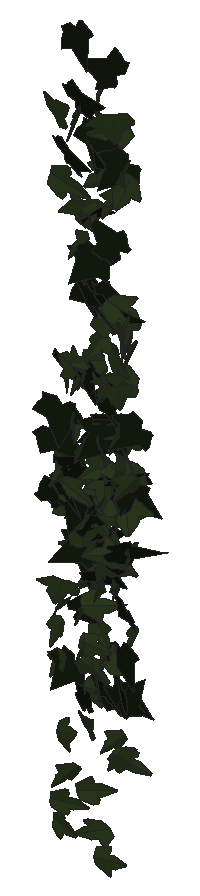
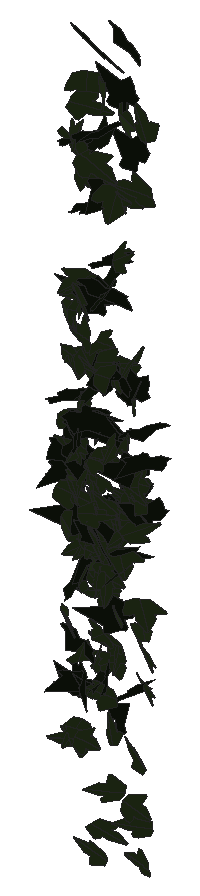
# SketchUp Ruby script. Lengths in inches.
U = 1.inch
M = Sketchup.active_model
def pt(a) = Geom::Point3d.new(a.map { |v| v * U })
def face(e, loops, mat)
  f = e.add_face(loops[0].map { |a| pt(a) })
  loops[1..].each { |l| e.add_face(l.map { |a| pt(a) }).erase! }
  f.material = f.back_material = mat if mat
  f
end
# faces: each face lists its corners as indices into pts; further lists are holes
def faces(e, pts, list, mat = nil) = list.each { |f| face(e, (f[0].is_a?(Array) ? f : [f]).map { |l| l.map { |i| pts[i] } }, mat) }
# xy, xz, yz: faces in a plane at the given z, y or x. An outline is a flat list of corners, or four numbers for a rectangle; further outlines are holes
def ring(l) = l.size == 4 ? [[l[0], l[1]], [l[2], l[1]], [l[2], l[3]], [l[0], l[3]]] : l.each_slice(2).to_a
def flat(e, list, mat, &to3) = list.each { |f| face(e, (f[0].is_a?(Array) ? f : [f]).map { |l| ring(l).map { |u, v| to3.(u, v) } }, mat) }
def xy(e, z, list, mat = nil) = flat(e, list, mat) { |x, y| [x, y, z] }
def xz(e, y, list, mat = nil) = flat(e, list, mat) { |x, z| [x, y, z] }
def yz(e, x, list, mat = nil) = flat(e, list, mat) { |y, z| [x, y, z] }
def lines(e, pts, list) = list.each { |a, b| e.add_line(pt(pts[a]), pt(pts[b])) }
# prism: a flat outline (further loops are holes) pulled along v
def prism(e, loops, v, mat = nil)
  f = face(e, loops, mat); d = Geom::Vector3d.new(v.map { |x| x * U })
  f.pushpull(f.normal.samedirection?(d) ? d.length : -d.length)
end
def box(e, o, s, mat = nil) = prism(e, [[o, [o[0] + s[0], o[1], o[2]], [o[0] + s[0], o[1] + s[1], o[2]], [o[0], o[1] + s[1], o[2]]]], [0, 0, s[2]], mat)
def at(x, y, z, deg = 0) = Geom::Transformation.translation(pt([x, y, z])) * Geom::Transformation.rotation(ORIGIN, Z_AXIS, deg.degrees)
def axes(o, x, y, z) = Geom::Transformation.new([*x, 0, *y, 0, *z, 0, *pt(o).to_a, 1])
def part(name) = M.definitions.add(name)
# library, detail: a bought-in or finely detailed component or shape, given as its bounding box
def library(name, o, s) = part(name).tap { |d| box(d.entities, o, s) }
def detail(e, o, s) = box(e.add_group.entities, o, s)
def put(e, d, t, mat = nil) = e.add_instance(d, t).tap { |i| i.material = mat if mat }
def group(e, t, mat = nil) = e.add_group.tap { |g| g.transformation = t; g.material = mat if mat }.entities
root = M.entities
M.materials.add("1026 AP 7946 SUNNY SIDE UP").color = [254, 231, 186]
M.materials.add("efeu1").color = [18, 25, 13]
M.materials.add("efeu2").color = [43, 57, 29]
c1 = part("ivyleaf_9")
p = [[1.54,2.16,1.25],[1.36,2.04,1.19],[-0.21,0.99,0.68],[-0.71,1.11,0.82],[-0.85,0.86,0.67],[-0.8,0.17,0.21],
  [-0.9,-0.01,0.1],[-0.67,-0.16,-0.02],[-0.08,-0.08,-0.05],[-0.03,-0.6,-0.4],[0.65,-0.88,-0.66],[0.83,-0.6,-0.49],
  [1.29,-0.42,-0.43],[1.8125,-0.07,-0.26],[1.21,0.44,0.15]]
faces(c1.entities,p,[[0,1,2,3,4,5,6,7,8,9,10,11,12,13,14]],"efeu1")
c2 = part("ivyleaf_10")
p = [[0,0.5,-0.03],[-0.0625,2.02,-0.43],[-0.19,2.01,-0.46],[-0.54,1.05,-0.29],[-0.52,0.625,-0.18],[-0.83,0.76,-0.28],
  [-1.16,0.64,-0.33],[-1.15,0.33,-0.24],[-0.77,-0.39,0.02],[-0.3,-0.51,0.16],[0.04,-0.48,0.23],[-0.02,2.01,-0.4375],
  [-0.06,2.01,-0.43],[0.04,-0.49,0.23],[0.67,-0.49,0.14],[1.38,0.36,-0.2],[1.375,0.51,-0.24],[0.81,0.65,-0.19],
  [0.62,0.59,-0.15],[0.6,1.09,-0.28],[0.5,1.23,-0.31]]
faces(c2.entities,p,[[0,1,2,3,4,5,6,7,8,9,10],[11,12,0,13,14,15,16,17,18,19,20]],"efeu2")
put(root,c1,axes([107.74,211.86,263.57],[-0.21606,-0.2106,0.03101],[0.02924,0.02523,0.2592],[-0.3335,0.13865,0.00264]),"1026 AP 7946 SUNNY SIDE UP")
put(root,c2,axes([107.53,211.98,256.62],[-0.01875,0.06088,0.24882],[-0.08228,-0.23667,0.0575],[0.38237,-0.04794,0.02457]),"1026 AP 7946 SUNNY SIDE UP")
put(root,c1,axes([106.36,211.97,265.17],[0.081,-0.09394,0.2637],[0.18372,-0.22836,-0.11166],[0.38825,0.12766,-0.00217]),"1026 AP 7946 SUNNY SIDE UP")
put(root,c2,axes([108.03,211.95,258.46],[-0.08063,-0.18421,0.15108],[-0.04481,-0.14521,-0.19761],[0.36854,-0.05796,0.00903]),"1026 AP 7946 SUNNY SIDE UP")
put(root,c2,axes([107.375,211.77,259.1],[-0.17753,0.19137,0.03851],[-0.04168,0.02647,-0.22855],[-0.30342,-0.1156,0.00886]),"1026 AP 7946 SUNNY SIDE UP")
put(root,c2,axes([107.32,211.89,249.84],[0.05886,-0.03965,-0.22419],[0.30721,-0.09708,0.05233],[-0.16234,-0.19808,0.01775]),"1026 AP 7946 SUNNY SIDE UP")
put(root,c2,axes([106.58,211.9375,260.52],[-0.06572,0.19876,0.16142],[0.04374,-0.15309,0.20832],[0.39445,0.05009,0.00379]),"1026 AP 7946 SUNNY SIDE UP")
put(root,c2,axes([106.3,212.04,258.17],[0.00091,-0.09245,0.25829],[0.10621,-0.24307,-0.09373],[0.40734,0.06358,0.02386]),"1026 AP 7946 SUNNY SIDE UP")
put(root,c1,axes([106.26,211.89,257.89],[0.22774,-0.20459,-0.01721],[-0.03157,0.0048,-0.25783],[0.32108,0.14559,-0.01315]),"1026 AP 7946 SUNNY SIDE UP")
put(root,c2,axes([107.92,211.75,252.375],[-0.13572,-0.16627,-0.15928],[0.12601,0.13137,-0.19205],[0.33296,-0.11749,0.00776]),"1026 AP 7946 SUNNY SIDE UP")
put(root,c2,axes([106.99,211.84,254.1],[-0.22026,0.00552,-0.16266],[0.24491,-0.03082,-0.14361],[-0.04196,-0.20884,0.01565]),"1026 AP 7946 SUNNY SIDE UP")
put(root,c2,axes([106.22,211.95,255.01],[-0.03371,-0.18183,-0.10836],[0.03224,-0.10602,0.1857],[-0.32791,0.00827,0.0294]),"1026 AP 7946 SUNNY SIDE UP")
put(root,c2,axes([107.8125,211.76,259.49],[0.04087,-0.20843,-0.15034],[0.05864,0.14706,-0.2104],[0.39468,-0.00027,0.04683]),"1026 AP 7946 SUNNY SIDE UP")
put(root,c1,axes([107.78,212.03,255.5],[0.21771,-0.15083,-0.14027],[0.16893,-0.08429,0.20958],[-0.27013,-0.17428,0.01802]),"1026 AP 7946 SUNNY SIDE UP")
put(root,c2,axes([106.95,211.89,254.51],[-0.01203,-0.04014,-0.2069],[0.3012,-0.07192,0.00688],[-0.113,-0.18743,0.04036]),"1026 AP 7946 SUNNY SIDE UP")
put(root,c2,axes([107.33,211.9,250.46],[0.18614,0.00012,-0.18652],[-0.28389,-0.01608,-0.12172],[-0.02127,0.21572,-0.0077]),"1026 AP 7946 SUNNY SIDE UP")
put(root,c2,axes([106.84,211.96,255.31],[0.11938,-0.17135,0.0987],[0.04413,-0.09324,-0.19331],[0.30628,0.08023,-0.01062]),"1026 AP 7946 SUNNY SIDE UP")
put(root,c2,axes([107.76,211.85,260.45],[-0.22263,-0.1791,-0.02998],[0.04517,0.01303,-0.23466],[0.28146,-0.14376,0.01394]),"1026 AP 7946 SUNNY SIDE UP")
put(root,c2,axes([106.73,212.03,260.33],[0.02798,-0.09098,0.2106],[0.1029,-0.19453,-0.09596],[0.33723,0.0669,0.01181]),"1026 AP 7946 SUNNY SIDE UP")
put(root,c1,axes([106.74,211.96,257.64],[-0.33813,-0.04783,-0.13158],[0.20332,0.00276,-0.2258],[0.06695,-0.24996,0.02117]),"1026 AP 7946 SUNNY SIDE UP")
put(root,c2,axes([106.21,211.93,254.66],[0.25447,-0.16877,0.03576],[0.02379,-0.03484,-0.24072],[0.2702,0.16202,-0.01248]),"1026 AP 7946 SUNNY SIDE UP")
put(root,c2,axes([106.26,211.99,252.24],[0.10331,-0.09168,-0.22143],[0.21561,-0.16501,0.115],[-0.2966,-0.15188,0.00647]),"1026 AP 7946 SUNNY SIDE UP")
put(root,c2,axes([107.14,211.76,255.48],[0.08102,-0.03015,-0.23432],[0.32054,0.11262,0.03288],[0.16496,-0.20403,0.05119]),"1026 AP 7946 SUNNY SIDE UP")
put(root,c2,axes([106.26,211.91,253.94],[0.24718,-0.15383,-0.00237],[-0.01739,-0.00926,-0.22615],[0.24126,0.15693,-0.01387]),"1026 AP 7946 SUNNY SIDE UP")
put(root,c1,axes([106.83,212.05,256.52],[-0.23879,-0.12122,0.16412],[-0.17551,-0.11575,-0.20017],[0.26233,-0.18778,0.01547]),"1026 AP 7946 SUNNY SIDE UP")
put(root,c1,axes([107.5,212.02,259.33],[-0.39822,-0.10606,0.02774],[-0.02397,-0.03455,-0.2818],[0.17062,-0.25239,0.02516]),"1026 AP 7946 SUNNY SIDE UP")
put(root,c2,axes([107.53,211.77,256.5],[-0.09433,-0.14775,-0.19472],[0.1714,0.15581,-0.16093],[0.33488,-0.12137,0.02752]),"1026 AP 7946 SUNNY SIDE UP")
put(root,c2,axes([107.05,211.8,264.07],[0.17883,0.00754,0.22406],[-0.32579,0.07865,0.10929],[-0.10444,-0.23245,0.04273]),"1026 AP 7946 SUNNY SIDE UP")
put(root,c1,axes([106.4375,211.84,258.27],[0.22114,0.0043,0.20837],[0.31437,-0.04039,-0.14259],[0.04834,0.243,-0.02592]),"1026 AP 7946 SUNNY SIDE UP")
put(root,c1,axes([106.2,212.04,259.46],[-0.13456,-0.25682,-0.00023],[0.01779,-0.00507,-0.27861],[0.40343,-0.08543,0.01221]),"1026 AP 7946 SUNNY SIDE UP")
put(root,c2,axes([106.45,211.87,257.85],[0.15153,0.04384,0.20203],[0.29469,0.05809,-0.10805],[-0.11293,0.21041,-0.01088]),"1026 AP 7946 SUNNY SIDE UP")
put(root,c2,axes([106.3,211.92,255.59],[-0.32208,-0.10863,0.05832],[-0.05914,-0.05045,-0.23763],[0.18379,-0.2066,0.02574]),"1026 AP 7946 SUNNY SIDE UP")
put(root,c2,axes([107.61,211.9,266.42],[-0.29512,-0.21512,-0.0242],[0.04752,0.00311,-0.29332],[0.33672,-0.18898,0.02018]),"1026 AP 7946 SUNNY SIDE UP")
put(root,c1,axes([106.93,211.94,262.39],[0.26374,-0.22877,-0.03467],[-0.04034,0.02129,-0.29199],[0.36105,0.16949,-0.0073]),"1026 AP 7946 SUNNY SIDE UP")
put(root,c1,axes([107.78,211.75,256.88],[0.12162,0.15281,-0.2031],[0.11526,0.18432,0.17711],[0.37602,-0.10592,0.0114]),"1026 AP 7946 SUNNY SIDE UP")
put(root,c2,axes([107.87,211.96,265.07],[0.41638,-0.1053,0.00529],[-0.00698,-0.02661,-0.29248],[0.16568,0.26353,-0.02561]),"1026 AP 7946 SUNNY SIDE UP")
put(root,c1,axes([107.3,211.75,256.26],[0.29322,0.16969,0.06102],[0.0868,0.0257,-0.25895],[-0.26843,0.19367,-0.01708]),"1026 AP 7946 SUNNY SIDE UP")
put(root,c1,axes([106.43,212.11,253.76],[-0.1557,-0.1891,0.14242],[-0.08489,-0.12882,-0.22041],[0.35943,-0.11234,0.00963]),"1026 AP 7946 SUNNY SIDE UP")
put(root,c2,axes([107.67,211.97,261.75],[-0.17446,0.19419,-0.14016],[0.09087,-0.12479,-0.23091],[-0.36262,-0.1247,0.00957]),"1026 AP 7946 SUNNY SIDE UP")
put(root,c2,axes([107.01,211.77,251.28],[-0.03202,-0.01537,0.23759],[0.1758,0.20208,0.02522],[-0.31826,0.11317,-0.00997]),"1026 AP 7946 SUNNY SIDE UP")
put(root,c2,axes([107.31,211.89,256.66],[-0.31033,-0.0945,-0.0801],[0.12718,0.00866,-0.22383],[0.1437,-0.21175,0.02511]),"1026 AP 7946 SUNNY SIDE UP")
put(root,c2,axes([106.29,211.83,250.79],[0.0159,0.00125,0.21883],[0.26163,0.13214,-0.00819],[-0.20762,0.16661,0.00644]),"1026 AP 7946 SUNNY SIDE UP")
put(root,c2,axes([107.76,212.12,265.1875],[0.00812,-0.02825,-0.26963],[0.00232,-0.26161,0.02761],[-0.41367,-0.00202,-0.00514]),"1026 AP 7946 SUNNY SIDE UP")
put(root,c2,axes([107.01,211.94,257.18],[-0.3478,-0.09654,0.06634],[-0.07875,-0.04691,-0.24785],[0.16513,-0.2257,0.02152]),"1026 AP 7946 SUNNY SIDE UP")
put(root,c2,axes([107.62,212.06,260.47],[-0.06684,-0.17088,0.17224],[-0.0611,-0.16362,-0.18236],[0.372,-0.05757,0.001]),"1026 AP 7946 SUNNY SIDE UP")
put(root,c2,axes([106.9375,211.87,257.56],[0.13867,-0.19963,-0.12073],[-0.05588,0.11102,-0.2239],[0.35877,0.09445,0.01179]),"1026 AP 7946 SUNNY SIDE UP")
put(root,c2,axes([106.61,211.96,257.34],[-0.16438,-0.02586,-0.18626],[0.27686,-0.06904,-0.09519],[-0.07546,-0.19697,0.05651]),"1026 AP 7946 SUNNY SIDE UP")
put(root,c2,axes([106.92,211.98,252.54],[-0.23824,0.10089,0.12077],[0.16252,-0.05496,0.18693],[0.17999,0.18315,-0.00894]),"1026 AP 7946 SUNNY SIDE UP")
put(root,c2,axes([107.25,212.0625,258.51],[0.14223,0.08095,-0.21896],[-0.20322,-0.17052,-0.1243],[-0.29509,0.15645,-0.01994]),"1026 AP 7946 SUNNY SIDE UP")
put(root,c1,axes([106.98,212.09,253.88],[0.07345,-0.04584,-0.24702],[0.33462,-0.11143,0.06408],[-0.18726,-0.2171,0.01761]),"1026 AP 7946 SUNNY SIDE UP")
put(root,c1,axes([107.19,211.95,253.77],[0.22996,-0.18535,-0.06762],[-0.07722,0.04342,-0.2427],[0.29881,0.15386,-0.01068]),"1026 AP 7946 SUNNY SIDE UP")
put(root,c1,axes([108.07,212.12,259.57],[-0.23159,-0.15216,0.12236],[-0.11148,-0.09748,-0.21821],[0.28321,-0.1628,0.01417]),"1026 AP 7946 SUNNY SIDE UP")
put(root,c1,axes([106.58,212.05,266.4],[0.02976,-0.03152,0.26823],[0.22501,-0.21774,-0.03912],[0.34593,0.14434,0.00237]),"1026 AP 7946 SUNNY SIDE UP")
put(root,c2,axes([107.85,211.95,257.86],[0.33833,0.17144,0.02198],[0.04393,-0.00247,-0.28274],[-0.26789,0.21611,-0.01861]),"1026 AP 7946 SUNNY SIDE UP")
put(root,c2,axes([107.4,211.84,261.92],[-0.05483,-0.07912,-0.25567],[0.35769,0.11186,-0.06914],[0.19818,-0.22378,0.05404]),"1026 AP 7946 SUNNY SIDE UP")
put(root,c2,axes([108.01,212,261.41],[0.11432,-0.22055,0.03662],[0.00036,-0.03862,-0.23916],[0.35159,0.07175,-0.01166]),"1026 AP 7946 SUNNY SIDE UP")
put(root,c2,axes([107.75,211.93,252.22],[-0.13769,-0.02631,-0.22511],[0.34578,-0.01461,-0.08912],[-0.00608,-0.23481,0.02937]),"1026 AP 7946 SUNNY SIDE UP")
put(root,c2,axes([106.88,211.92,264.23],[-0.34232,-0.18338,-0.06204],[0.09201,0.02215,-0.29237],[0.28869,-0.22452,0.01962]),"1026 AP 7946 SUNNY SIDE UP")
put(root,c2,axes([107.52,212.03,260.55],[-0.11296,-0.25327,0.09023],[-0.02988,-0.08712,-0.27167],[0.42107,-0.07413,0.00493]),"1026 AP 7946 SUNNY SIDE UP")
put(root,c2,axes([107.74,212.05,257.67],[0.06659,-0.20674,0.09492],[0.04886,-0.08874,-0.2176],[0.3533,0.05124,0.01221]),"1026 AP 7946 SUNNY SIDE UP")
put(root,c2,axes([106.55,212.12,266.09],[0.1478,-0.18233,0.18788],[0.11166,-0.16945,-0.21202],[0.39102,0.1173,-0.01047]),"1026 AP 7946 SUNNY SIDE UP")
put(root,c2,axes([107.22,212.09,258.49],[-0.09728,-0.15888,0.16128],[-0.02006,-0.1606,-0.17305],[0.35116,-0.05319,0.03479]),"1026 AP 7946 SUNNY SIDE UP")
put(root,c1,axes([107.125,212.16,265.3],[-0.09978,-0.10564,0.23131],[0.02548,-0.2336,-0.10959],[0.39019,-0.01176,0.06631]),"1026 AP 7946 SUNNY SIDE UP")
put(root,c2,axes([107.29,211.85,255.93],[0.04552,-0.1647,-0.18394],[0.01513,0.17952,-0.16882],[0.38058,0.01256,0.02872]),"1026 AP 7946 SUNNY SIDE UP")
put(root,c2,axes([106.9,211.86,258.875],[-0.04802,-0.16481,-0.1778],[0.09552,0.16193,-0.17036],[0.36179,-0.06463,0.02138]),"1026 AP 7946 SUNNY SIDE UP")
put(root,c2,axes([107.18,212.11,256.06],[-0.10128,-0.12152,0.2007],[-0.12641,-0.17835,-0.14254],[0.33917,-0.10276,0.0068]),"1026 AP 7946 SUNNY SIDE UP")
put(root,c2,axes([106.75,211.79,256.93],[0.01613,0.05069,0.24878],[-0.04803,0.23981,-0.04918],[-0.38457,-0.02783,0.01658]),"1026 AP 7946 SUNNY SIDE UP")
put(root,c1,axes([107.24,212.05,260],[0.18751,-0.22309,-0.0033],[-0.01818,-0.00399,-0.26033],[0.35034,0.1192,-0.01174]),"1026 AP 7946 SUNNY SIDE UP")
put(root,c2,axes([107.77,212.15,261.52],[-0.01324,-0.1223,0.22775],[0.17348,-0.2015,-0.11134],[0.35845,0.093,0.0623]),"1026 AP 7946 SUNNY SIDE UP")
put(root,c2,axes([107.19,212.13,254.15],[-0.02463,0.00394,0.22355],[0.17691,-0.18587,0.01076],[0.29179,0.11302,0.01235]),"1026 AP 7946 SUNNY SIDE UP")
put(root,c2,axes([106.85,211.89,254.375],[0.01257,-0.14857,-0.1449],[0.01916,0.14001,-0.15175],[0.32021,-0.00255,0.01477]),"1026 AP 7946 SUNNY SIDE UP")
put(root,c1,axes([107.16,211.79,264.17],[0.15366,0.18175,0.13927],[0.09901,0.11846,-0.2119],[-0.34113,0.11625,0.00124]),"1026 AP 7946 SUNNY SIDE UP")
put(root,c2,axes([106.73,212.02,256.58],[-0.27484,-0.14306,0.03878],[-0.0302,-0.03709,-0.2323],[0.23096,-0.17508,0.01577]),"1026 AP 7946 SUNNY SIDE UP")
put(root,c2,axes([107.44,212.11,261.01],[0.06055,-0.0496,0.26709],[0.36903,-0.1141,-0.059],[0.19092,0.23628,0.02934]),"1026 AP 7946 SUNNY SIDE UP")
put(root,c2,axes([107.96,212.1,256.89],[0.07417,-0.19848,0.10478],[0.05271,-0.09763,-0.21054],[0.34752,0.05717,0.00957]),"1026 AP 7946 SUNNY SIDE UP")
put(root,c1,axes([107.93,211.96,258.48],[0.0805,0.22744,-0.11678],[-0.03033,-0.11314,-0.24077],[-0.39935,0.05444,-0.00525]),"1026 AP 7946 SUNNY SIDE UP")
put(root,c2,axes([106.46,212.15,257.86],[0.04014,0.02587,-0.22513],[-0.21933,-0.16844,-0.03829],[-0.26792,0.14177,-0.00239]),"1026 AP 7946 SUNNY SIDE UP")
put(root,c1,axes([106.125,211.85,257.47],[-0.08987,-0.00873,0.26578],[0.34043,0.14237,0.05519],[-0.22119,0.22267,-0.02303]),"1026 AP 7946 SUNNY SIDE UP")
put(root,c2,axes([106.09,212.0625,250.13],[0.01711,0.01795,0.21627],[0.32365,-0.04535,-0.00726],[0.07005,0.20516,-0.01926]),"1026 AP 7946 SUNNY SIDE UP")
put(root,c2,axes([106.12,212.02,264.53],[0.06617,0.02065,0.27736],[0.42195,0.02602,-0.04513],[-0.04554,0.27114,-0.01519]),"1026 AP 7946 SUNNY SIDE UP")
put(root,c2,axes([107.5,212.15,264.59],[-0.03745,-0.20378,0.15586],[0.02207,-0.15394,-0.21062],[0.39956,-0.0106,0.02624]),"1026 AP 7946 SUNNY SIDE UP")
put(root,c2,axes([107.01,212.03,253.45],[-0.00687,-0.01707,-0.25444],[0.38236,-0.04619,-0.00141],[-0.07232,-0.24257,0.0167]),"1026 AP 7946 SUNNY SIDE UP")
put(root,c2,axes([106.38,212.15,251.37],[-0.05609,-0.15665,0.16399],[-0.06098,-0.15532,-0.1664],[0.34685,-0.05264,-0.00274]),"1026 AP 7946 SUNNY SIDE UP")
put(root,c1,axes([107.48,212.11,259.24],[0.05424,0.03059,-0.26161],[-0.18828,-0.22469,-0.04592],[-0.3557,0.1236,-0.01559]),"1026 AP 7946 SUNNY SIDE UP")
put(root,c1,axes([106.25,212.17,260.23],[-0.06792,-0.06134,0.2565],[0.17471,-0.2324,-0.04043],[0.36398,0.10011,0.06727]),"1026 AP 7946 SUNNY SIDE UP")
put(root,c1,axes([107.1,212.07,256.84],[0.29748,0.06186,0.15449],[-0.23667,-0.01753,0.20345],[0.09374,-0.24056,0.02339]),"1026 AP 7946 SUNNY SIDE UP")
put(root,c2,axes([107.2,212.08,258.1],[0.34342,-0.05256,0.07836],[0.10714,-0.04152,-0.23044],[0.09885,0.22762,-0.02249]),"1026 AP 7946 SUNNY SIDE UP")
put(root,c2,axes([106.99,212.16,260.7],[0.06252,0.01384,-0.24319],[-0.28624,-0.15111,-0.04159],[-0.2375,0.18576,-0.0139]),"1026 AP 7946 SUNNY SIDE UP")
put(root,c1,axes([106.64,212.125,260.52],[-0.09555,-0.03351,-0.25754],[0.396,-0.01822,-0.0607],[-0.01564,-0.25644,0.03644]),"1026 AP 7946 SUNNY SIDE UP")
put(root,c1,axes([107.64,212.1,254.49],[-0.17287,-0.03478,-0.2319],[0.35383,0.02073,-0.1165],[0.05349,-0.24948,0.02115]),"1026 AP 7946 SUNNY SIDE UP")
put(root,c2,axes([107.53,211.98,256.53],[-0.20111,-0.08469,-0.16297],[0.2419,0.04713,-0.15432],[0.14395,-0.19752,0.03163]),"1026 AP 7946 SUNNY SIDE UP")
put(root,c1,axes([106.93,212.23,262.92],[-0.22422,-0.18002,0.12443],[-0.09261,-0.10822,-0.23644],[0.32897,-0.15316,0.01824]),"1026 AP 7946 SUNNY SIDE UP")
put(root,c1,axes([107.68,212.22,265.29],[-0.24292,-0.17564,0.10536],[-0.08704,-0.08854,-0.24097],[0.30832,-0.16338,0.01498]),"1026 AP 7946 SUNNY SIDE UP")
put(root,c1,axes([106.04,212.01,258.87],[0.02521,-0.17472,-0.20043],[0.07592,0.19256,-0.17382],[0.40293,-0.02535,0.04529]),"1026 AP 7946 SUNNY SIDE UP")
put(root,c2,axes([106.02,212.11,265.9],[-0.29898,0.0969,0.17714],[0.25772,-0.05414,0.21853],[0.17156,0.2502,-0.01957]),"1026 AP 7946 SUNNY SIDE UP")
put(root,c1,axes([106.84,212.16,260.375],[0.3133,-0.04719,-0.17033],[0.25991,-0.01563,0.21005],[-0.07297,-0.25827,0.01685]),"1026 AP 7946 SUNNY SIDE UP")
put(root,c1,axes([107.11,212.08,261.89],[0.12818,-0.02631,0.25199],[0.32631,-0.13132,-0.08651],[0.20818,0.22204,-0.01954]),"1026 AP 7946 SUNNY SIDE UP")
put(root,c1,axes([106.75,211.93,255.14],[0.0856,0.04674,0.24187],[0.35965,0.05999,-0.06666],[-0.1097,0.23316,-0.02983]),"1026 AP 7946 SUNNY SIDE UP")
put(root,c1,axes([107.6875,211.99,253.3],[-0.22507,0.06926,0.1897],[0.27554,-0.05756,0.16264],[0.13935,0.2257,-0.0152]),"1026 AP 7946 SUNNY SIDE UP")
put(root,c2,axes([107.8125,212.11,259.23],[-0.23702,-0.15564,0.07232],[-0.05226,-0.06629,-0.22254],[0.26392,-0.15291,0.02088]),"1026 AP 7946 SUNNY SIDE UP")
put(root,c2,axes([106.36,211.9375,258.21],[-0.10908,0.06203,-0.21239],[-0.19002,0.16848,0.09494],[0.2808,0.13811,-0.01826]),"1026 AP 7946 SUNNY SIDE UP")
put(root,c1,axes([107.75,211.96,253.73],[0.11665,-0.02249,-0.24708],[-0.3665,0.05615,-0.07941],[0.09488,0.24457,-0.00298]),"1026 AP 7946 SUNNY SIDE UP")
put(root,c2,axes([107.05,212.12,254.79],[0.22618,-0.02603,0.15435],[0.22594,-0.04488,-0.15026],[0.07899,0.2029,-0.01217]),"1026 AP 7946 SUNNY SIDE UP")
put(root,c2,axes([107.3,212.06,257.82],[0.03365,-0.21686,-0.05276],[0.00235,0.05036,-0.2241],[0.34992,0.02052,0.00658]),"1026 AP 7946 SUNNY SIDE UP")
put(root,c2,axes([107.59,212.18,266.05],[0.10936,0.05112,-0.24284],[-0.331,-0.10752,-0.08852],[-0.18607,0.22131,0.01475]),"1026 AP 7946 SUNNY SIDE UP")
put(root,c2,axes([107.72,211.9,258.63],[-0.00116,-0.12165,-0.26216],[0.07953,0.2496,-0.12195],[0.43533,-0.04592,0.02158]),"1026 AP 7946 SUNNY SIDE UP")
put(root,c2,axes([107.32,211.95,255.99],[0.10787,-0.09316,0.18404],[-0.11791,0.16395,0.11836],[-0.29484,-0.09965,0.02]),"1026 AP 7946 SUNNY SIDE UP")
put(root,c2,axes([107.13,212.13,256.77],[-0.23128,0.08801,-0.16744],[0.19299,-0.10965,-0.17569],[-0.21823,-0.19024,0.02208]),"1026 AP 7946 SUNNY SIDE UP")
put(root,c2,axes([107.44,212.24,255.83],[-0.05403,0.06235,0.23031],[0.1612,-0.19828,0.07216],[0.32681,0.10811,0.00249]),"1026 AP 7946 SUNNY SIDE UP")
put(root,c2,axes([106.32,212.2,257.23],[0.04894,0.13222,0.20945],[-0.13726,-0.18433,0.13669],[0.35473,-0.08956,0.024]),"1026 AP 7946 SUNNY SIDE UP")
put(root,c2,axes([107.9,212.12,258.62],[0.35081,-0.03227,-0.04394],[-0.06991,-0.01164,-0.23159],[0.04632,0.22681,-0.01678]),"1026 AP 7946 SUNNY SIDE UP")
put(root,c1,axes([106.59,212.25,256.28],[0.02385,-0.25276,0.08069],[0.00955,-0.07953,-0.26132],[0.41665,0.01629,0.00137]),"1026 AP 7946 SUNNY SIDE UP")
put(root,c2,axes([107.71,212.01,257.57],[0.13908,-0.20081,0.11885],[-0.04635,0.11396,0.22606],[-0.36211,-0.09172,0.01672]),"1026 AP 7946 SUNNY SIDE UP")
put(root,c1,axes([107.46,212.2,259.41],[0.03982,0.02445,-0.26121],[-0.15258,-0.23481,-0.03467],[-0.37057,0.09931,-0.01379]),"1026 AP 7946 SUNNY SIDE UP")
put(root,c2,axes([106.47,212.15,259.21],[-0.00841,0.19607,-0.11422],[-0.00585,-0.11208,-0.20263],[-0.355,-0.0028,0.00604]),"1026 AP 7946 SUNNY SIDE UP")
put(root,c1,axes([107.02,212.08,256.5625],[-0.05143,0.19897,0.14613],[0.03894,-0.13853,0.20691],[0.38122,0.041,-0.00142]),"1026 AP 7946 SUNNY SIDE UP")
put(root,c2,axes([107.58,211.97,262.22],[0.13604,0.16411,0.19056],[0.15424,0.15604,-0.18993],[-0.35573,0.13042,-0.00947]),"1026 AP 7946 SUNNY SIDE UP")
put(root,c2,axes([107.43,212.09,256.85],[0.24096,-0.19306,-0.09496],[-0.11059,0.0602,-0.253],[0.31692,0.16779,-0.01608]),"1026 AP 7946 SUNNY SIDE UP")
put(root,c2,axes([107.49,212.23,252.43],[-0.04405,-0.11727,0.17856],[-0.03023,-0.17337,-0.12458],[0.32855,-0.03168,0.01248]),"1026 AP 7946 SUNNY SIDE UP")
put(root,c1,axes([107.56,211.99,267.35],[-0.20591,0.17858,0.18446],[-0.19886,0.12705,-0.22637],[-0.34303,-0.18084,0.02051]),"1026 AP 7946 SUNNY SIDE UP")
put(root,c1,axes([107.67,212.28,258.67],[0.01084,-0.09875,0.25243],[0.06722,-0.24204,-0.10291],[0.41075,0.04222,0.01018]),"1026 AP 7946 SUNNY SIDE UP")
put(root,c1,axes([107.68,212.27,258.625],[-0.00139,-0.03507,0.26178],[0.0112,-0.25421,-0.03758],[0.4035,0.00693,0.00194]),"1026 AP 7946 SUNNY SIDE UP")
put(root,c2,axes([107.7,212.1,261.97],[0.23622,-0.21325,-0.07577],[-0.07568,0.05454,-0.26829],[0.34589,0.15757,-0.00696]),"1026 AP 7946 SUNNY SIDE UP")
put(root,c1,axes([107.55,212.04,253.61],[0.01007,-0.08753,-0.23414],[0.17982,0.20127,-0.07553],[0.33729,-0.10469,0.04726]),"1026 AP 7946 SUNNY SIDE UP")
put(root,c2,axes([107.56,212.03,258.02],[-0.12044,0.22685,0.0661],[-0.04549,0.05655,-0.24615],[-0.36734,-0.08138,0.00881]),"1026 AP 7946 SUNNY SIDE UP")
put(root,c1,axes([106.8,212.03,253.03],[0.07572,-0.09258,0.22915],[-0.07552,0.21913,0.10571],[-0.37202,-0.06333,0.02518]),"1026 AP 7946 SUNNY SIDE UP")
put(root,c2,axes([107.02,212.0625,255.97],[-0.06188,-0.22846,-0.09313],[0.01557,0.08869,-0.23825],[0.38526,-0.04028,-0.00533]),"1026 AP 7946 SUNNY SIDE UP")
put(root,c1,axes([106.95,212.32,262.09],[-0.01769,-0.16554,0.20505],[-0.02697,-0.19925,-0.17208],[0.40731,-0.02039,-0.00249]),"1026 AP 7946 SUNNY SIDE UP")
put(root,c1,axes([106.4,212.24,267.84],[-0.14177,-0.07782,-0.25642],[0.40929,-0.02092,-0.09068],[0.00938,-0.26349,0.08125]),"1026 AP 7946 SUNNY SIDE UP")
put(root,c2,axes([106.91,212.29,260.45],[-0.07996,-0.10956,0.22911],[-0.04206,-0.2239,-0.12091],[0.38844,-0.04679,0.03407]),"1026 AP 7946 SUNNY SIDE UP")
put(root,c2,axes([107.9,212.09,260.51],[-0.03478,0.07511,0.23358],[-0.37492,-0.00894,-0.02101],[0.00326,-0.22721,0.07657]),"1026 AP 7946 SUNNY SIDE UP")
put(root,c1,axes([106.98,212.28,265.7],[-0.10068,-0.27048,0.04403],[-0.00443,-0.04482,-0.2865],[0.43094,-0.06365,0.00734]),"1026 AP 7946 SUNNY SIDE UP")
put(root,c2,axes([106.16,212.28,260.2],[0.01731,-0.10873,0.23127],[0.2286,-0.18053,-0.09821],[0.3198,0.13493,0.05769]),"1026 AP 7946 SUNNY SIDE UP")
put(root,c2,axes([107.91,212.17,254.9375],[0.18213,-0.19221,0.02128],[0.00242,-0.02443,-0.23104],[0.30415,0.11529,-0.01091]),"1026 AP 7946 SUNNY SIDE UP")
put(root,c1,axes([107.88,212.01,258.11],[0.0248,-0.0817,-0.23768],[0.01113,0.23078,-0.08251],[0.384,-0.00141,0.01774]),"1026 AP 7946 SUNNY SIDE UP")
put(root,c2,axes([106.52,212.3125,263.11],[0.00422,-0.03407,0.25438],[0.10645,-0.23776,-0.03591],[0.37753,0.06742,0.00728]),"1026 AP 7946 SUNNY SIDE UP")
put(root,c2,axes([107.6,212.08,254.08],[0.1135,0.20689,-0.01008],[-0.00479,0.01267,0.22569],[0.32573,-0.0719,0.00683]),"1026 AP 7946 SUNNY SIDE UP")
put(root,c2,axes([106.9,212.32,266.46],[-0.02275,0.01317,-0.2721],[0.0772,-0.25987,-0.01764],[-0.40872,-0.04981,0.01181]),"1026 AP 7946 SUNNY SIDE UP")
put(root,c2,axes([106.14,212.2,257.98],[-0.03879,-0.04039,-0.24697],[0.33608,-0.11796,-0.00288],[-0.18141,-0.20989,0.04748]),"1026 AP 7946 SUNNY SIDE UP")
put(root,c2,axes([107.03,212.24,261.16],[0.08847,0.13145,-0.17738],[-0.09969,-0.16091,-0.14821],[-0.32668,0.08471,-0.00281]),"1026 AP 7946 SUNNY SIDE UP")
put(root,c2,axes([107.33,212.26,257.33],[-0.01894,0.02172,0.23326],[-0.18257,-0.19542,0.01181],[0.30733,-0.11475,0.02139]),"1026 AP 7946 SUNNY SIDE UP")
put(root,c2,axes([106.86,212.11,257.55],[0.25118,-0.05226,-0.15282],[0.23908,-0.00113,0.16942],[-0.06151,-0.21779,0.03444]),"1026 AP 7946 SUNNY SIDE UP")
put(root,c1,axes([106.94,212.2,262.29],[-0.24952,-0.11937,-0.20194],[0.28028,0.08472,-0.20201],[0.22588,-0.23699,0.02758]),"1026 AP 7946 SUNNY SIDE UP")
put(root,c2,axes([107.32,212.23,264.93],[-0.22415,-0.09968,0.19898],[-0.22616,-0.13082,-0.17915],[0.25729,-0.20183,0.01588]),"1026 AP 7946 SUNNY SIDE UP")
put(root,c2,axes([107.85,212.25,257.65],[-0.12789,-0.05522,0.24382],[-0.27288,-0.16199,-0.10119],[0.2682,-0.19115,0.01331]),"1026 AP 7946 SUNNY SIDE UP")
